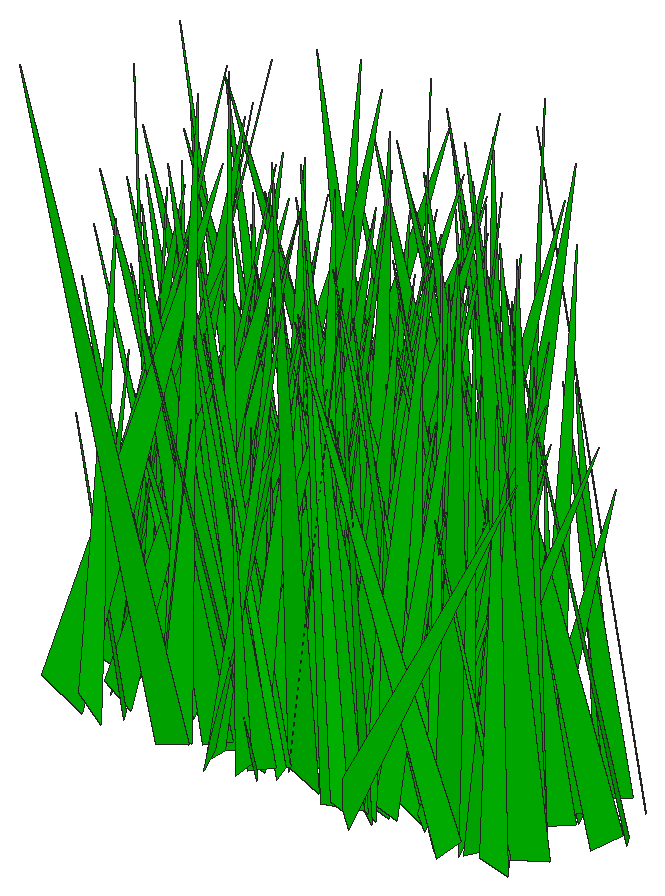
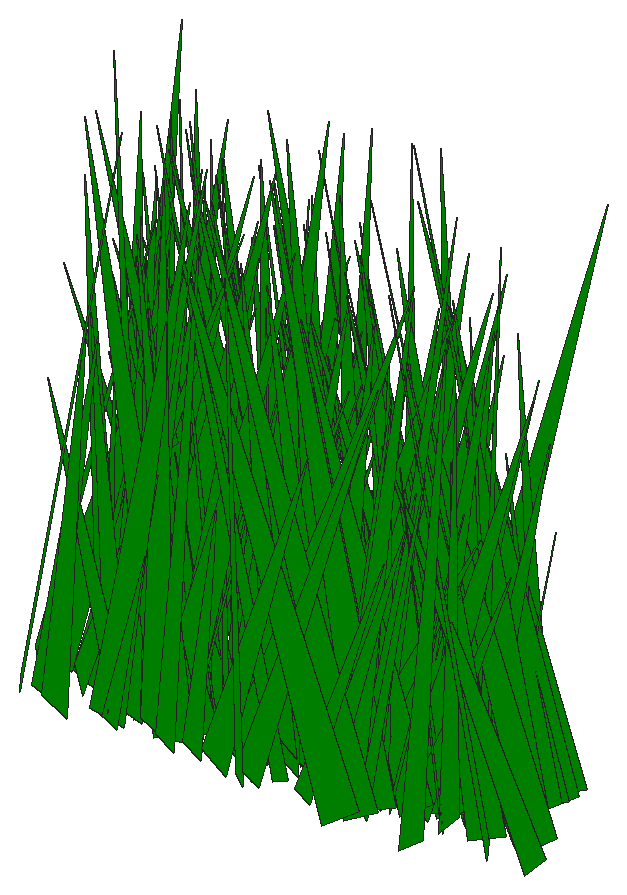
# SketchUp Ruby script. Lengths in inches.
U = 1.inch
M = Sketchup.active_model
def pt(a) = Geom::Point3d.new(a.map { |v| v * U })
def face(e, loops, mat)
  f = e.add_face(loops[0].map { |a| pt(a) })
  loops[1..].each { |l| e.add_face(l.map { |a| pt(a) }).erase! }
  f.material = f.back_material = mat if mat
  f
end
# faces: each face lists its corners as indices into pts; further lists are holes
def faces(e, pts, list, mat = nil) = list.each { |f| face(e, (f[0].is_a?(Array) ? f : [f]).map { |l| l.map { |i| pts[i] } }, mat) }
# xy, xz, yz: faces in a plane at the given z, y or x. An outline is a flat list of corners, or four numbers for a rectangle; further outlines are holes
def ring(l) = l.size == 4 ? [[l[0], l[1]], [l[2], l[1]], [l[2], l[3]], [l[0], l[3]]] : l.each_slice(2).to_a
def flat(e, list, mat, &to3) = list.each { |f| face(e, (f[0].is_a?(Array) ? f : [f]).map { |l| ring(l).map { |u, v| to3.(u, v) } }, mat) }
def xy(e, z, list, mat = nil) = flat(e, list, mat) { |x, y| [x, y, z] }
def xz(e, y, list, mat = nil) = flat(e, list, mat) { |x, z| [x, y, z] }
def yz(e, x, list, mat = nil) = flat(e, list, mat) { |y, z| [x, y, z] }
def lines(e, pts, list) = list.each { |a, b| e.add_line(pt(pts[a]), pt(pts[b])) }
# prism: a flat outline (further loops are holes) pulled along v
def prism(e, loops, v, mat = nil)
  f = face(e, loops, mat); d = Geom::Vector3d.new(v.map { |x| x * U })
  f.pushpull(f.normal.samedirection?(d) ? d.length : -d.length)
end
def box(e, o, s, mat = nil) = prism(e, [[o, [o[0] + s[0], o[1], o[2]], [o[0] + s[0], o[1] + s[1], o[2]], [o[0], o[1] + s[1], o[2]]]], [0, 0, s[2]], mat)
def at(x, y, z, deg = 0) = Geom::Transformation.translation(pt([x, y, z])) * Geom::Transformation.rotation(ORIGIN, Z_AXIS, deg.degrees)
def axes(o, x, y, z) = Geom::Transformation.new([*x, 0, *y, 0, *z, 0, *pt(o).to_a, 1])
def part(name) = M.definitions.add(name)
# library, detail: a bought-in or finely detailed component or shape, given as its bounding box
def library(name, o, s) = part(name).tap { |d| box(d.entities, o, s) }
def detail(e, o, s) = box(e.add_group.entities, o, s)
def put(e, d, t, mat = nil) = e.add_instance(d, t).tap { |i| i.material = mat if mat }
def group(e, t, mat = nil) = e.add_group.tap { |g| g.transformation = t; g.material = mat if mat }.entities
root = M.entities
M.materials.add("[Color G06]").color = [0, 204, 0]
c1 = part("fur_instance\#9")
p = [[0.8125,0,1.79],[0.67,-0.02,1.48],[0,-0.11,0],[0,0.11,0]]
faces(c1.entities,p,[[0,1,2,3]])
put(root,c1,axes([26.27,17.6875,4.28],[1.77503,-0.43818,1.91924],[-2.78158,-0.30358,-2.21547],[-1.94577,0.03424,4.91795]),"[Color G06]")
put(root,c1,axes([25.45,18.56,4.28],[4.99824,-0.16607,3.33353],[-0.63671,-0.74948,-2.15665],[-2.44698,-0.1442,7.37031]),"[Color G06]")
put(root,c1,axes([22.9,19.63,4.28],[2.96113,-0.41722,0.08202],[-2.68322,-0.36541,2.85818],[1.32498,0.19245,5.60482]),"[Color G06]")
put(root,c1,axes([27.2,19.07,4.28],[-1.54116,-0.61948,0.49557],[-4.26601,0.19114,-2.18785],[-1.28316,0.10858,6.67853]),"[Color G06]")
put(root,c1,axes([25.84,19.31,4.28],[-3.96562,0.38661,0.70973],[2.43463,0.52909,-2.72106],[1.40878,0.17392,6.70031]),"[Color G06]")
put(root,c1,axes([26.89,19.16,4.28],[-0.52699,-0.39708,0.70176],[-2.58056,0.03503,-2.05172],[-1.29225,0.09198,3.811]),"[Color G06]")
put(root,c1,axes([26.34,16.33,4.28],[-2.62712,-0.05537,0.68032],[-0.51987,0.35151,-1.19773],[0.3076,0.12115,3.78609]),"[Color G06]")
put(root,c1,axes([24.11,18.14,4.28],[2.16447,-0.64237,0.1245],[-4.56425,-0.2972,1.09648],[0.62903,0.05391,7.52764]),"[Color G06]")
put(root,c1,axes([25.19,16.5,4.28],[2.70805,0.30168,0.39465],[2.03734,-0.37126,1.3736],[-0.77423,0.07826,4.99494]),"[Color G06]")
put(root,c1,axes([25.5,16.09,4.28],[-3.84473,0.4154,1.17109],[2.44382,0.51774,-3.17502],[1.87511,0.17699,6.53922]),"[Color G06]")
put(root,c1,axes([23.45,18.68,4.28],[1.02615,-0.6579,0.47878],[-4.28554,-0.11006,3.14436],[1.99903,0.10178,6.49515]),"[Color G06]")
put(root,c1,axes([25.9375,20.67,4.28],[-3.70608,-0.57537,0.03348],[-3.88339,0.4878,2.7732],[1.39454,-0.17071,7.8115]),"[Color G06]")
put(root,c1,axes([24.31,19.71,4.28],[5.31499,0.07245,1.13215],[0.31095,-0.72555,2.07305],[-0.86434,0.1845,7.70759]),"[Color G06]")
put(root,c1,axes([28.03,15.97,4.28],[-3.66144,-0.67876,0.62945],[-4.83462,0.49276,-1.77831],[-0.70484,0.14601,8.92792]),"[Color G06]")
put(root,c1,axes([24.46,16.68,4.28],[2.90062,0.34995,0.36701],[2.50236,-0.39305,-1.12379],[0.31088,-0.10142,5.62135]),"[Color G06]")
put(root,c1,axes([25.41,18.16,4.28],[4.49687,-0.17073,1.75021],[-0.85864,-0.62894,-2.11996],[-1.46053,-0.15592,6.63512]),"[Color G06]")
put(root,c1,axes([25.95,18.68,4.28],[-2.37703,0.33297,1.33662],[2.26974,0.354,-1.11387],[1.16179,-0.01033,4.91088]),"[Color G06]")
put(root,c1,axes([27.375,17.76,4.28],[-4.54947,0.06993,1.36749],[0.87654,0.56578,3.19006],[0.56601,-0.31406,6.05135]),"[Color G06]")
put(root,c1,axes([24.36,16.68,4.28],[-0.65487,0.62361,2.23704],[4.18524,0.17397,-2.83423],[2.1734,-0.1471,6.13181]),"[Color G06]")
put(root,c1,axes([24.71,19.24,4.28],[0.60019,-0.77466,1.03045],[-5.39528,-0.05427,2.333],[1.49261,0.11534,8.01866]),"[Color G06]")
put(root,c1,axes([27.54,19.47,4.28],[-3.42438,-0.0279,0.36076],[-0.25947,0.45943,-1.41956],[0.17601,0.13443,4.92626]),"[Color G06]")
put(root,c1,axes([27.3,18.77,4.28],[0.57422,-0.64696,1.14365],[-4.49813,-0.1069,-1.90191],[-1.37015,0.07981,6.72314]),"[Color G06]")
put(root,c1,axes([24.34,18.8,4.28],[5.95512,0.27848,0.16632],[1.93577,-0.81472,1.87956],[-0.50328,0.16146,9.19741]),"[Color G06]")
put(root,c1,axes([24.26,17.625,4.28],[6.10667,0.17875,1.03682],[1.38375,-0.84191,-1.53103],[-0.45797,-0.16026,9.19926]),"[Color G06]")
put(root,c1,axes([25.86,17.86,4.28],[-0.90875,0.42445,0.57821],[2.87881,0.13741,-1.48109],[1.06173,-0.00929,4.51077]),"[Color G06]")
put(root,c1,axes([25.3125,17.2,4.28],[4.16854,-0.06504,0.77961],[-0.33247,-0.57072,-1.49838],[-0.6157,-0.13215,6.08737]),"[Color G06]")
put(root,c1,axes([26.09,19.32,4.28],[3.48305,0.17186,0.95936],[0.89412,-0.46209,2.25788],[-1.06371,0.17432,5.03924]),"[Color G06]")
put(root,c1,axes([27.15,17.91,4.28],[0.74767,-0.67482,0.03349],[-4.74169,-0.10279,-1.45787],[-0.96737,-0.01774,7.17185]),"[Color G06]")
put(root,c1,axes([27.29,18.67,4.28],[-2.84415,0.12768,0.36978],[0.78047,0.37703,-1.5453],[0.53888,0.12779,4.18973]),"[Color G06]")
put(root,c1,axes([27.29,18.96,4.28],[-1.89683,0.24786,1.64054],[2.08615,0.23568,1.29742],[0.11065,-0.19454,3.66209]),"[Color G06]")
put(root,c1,axes([24.59,16.21,4.28],[1.58891,0.79693,0.09119],[5.46262,-0.20916,-2.6313],[1.68071,-0.07359,8.46598]),"[Color G06]")
put(root,c1,axes([27.9,20.11,4.28],[-3.23169,-0.19871,1.21615],[-1.60974,0.43256,-1.43578],[0.31872,0.16984,5.07973]),"[Color G06]")
put(root,c1,axes([28.99,19.22,4.28],[-2.38445,-0.35832,0.45863],[-2.29156,0.26532,-2.80061],[-1.20243,0.20493,4.42786]),"[Color G06]")
put(root,c1,axes([28.12,19.46,4.28],[-5.64134,0.17742,2.7107],[1.82193,0.76517,2.71669],[1.26048,-0.31196,8.20511]),"[Color G06]")
put(root,c1,axes([25.63,16.95,4.28],[0.79235,0.49285,1.91099],[3.49801,-0.03004,-2.34969],[1.37486,-0.20759,4.87689]),"[Color G06]")
put(root,c1,axes([25.97,18.42,4.28],[4.63417,0.36447,0.19802],[2.55297,-0.63785,1.40507],[-0.57557,0.10529,7.82664]),"[Color G06]")
put(root,c1,axes([29.33,18.28,4.28],[-2.13214,-0.67353,1.27137],[-4.75759,0.25263,-2.44774],[-1.19101,0.19658,7.5017]),"[Color G06]")
put(root,c1,axes([28.49,19.98,4.28],[-3.85908,0.46128,2.08467],[3.54398,0.53508,1.05359],[0.57302,-0.20275,7.52325]),"[Color G06]")
put(root,c1,axes([28.28,19.57,4.28],[-0.4187,-0.42172,1.40295],[-3.09522,0.02663,-1.14395],[-0.66858,0.14083,4.41739]),"[Color G06]")
put(root,c1,axes([28.8125,16.65,4.28],[-0.3633,0.51505,2.97986],[4.01401,-0.03894,1.86635],[-1.22694,-0.27991,5.22354]),"[Color G06]")
put(root,c1,axes([29.05,16.83,4.28],[-1.94836,-0.30928,0.6708],[-2.14021,0.22503,-1.96701],[-0.73499,0.1646,3.94953]),"[Color G06]")
put(root,c1,axes([28,19.26,4.28],[-2.98145,0.478,0.87276],[3.32316,0.42326,-1.27154],[1.02366,0.01814,6.6698]),"[Color G06]")
put(root,c1,axes([29.15,20.14,4.28],[-1.99478,0.35344,0.24427],[2.46487,0.2624,1.34803],[-0.61263,-0.09508,4.62832]),"[Color G06]")
put(root,c1,axes([28.37,17.39,4.28],[-1.54046,0.39655,2.3548],[3.25066,0.19165,1.04269],[0.05044,-0.24018,4.71993]),"[Color G06]")
put(root,c1,axes([26.62,19.12,4.28],[1.68588,-0.68116,1.21395],[-4.92058,-0.21702,1.27575],[0.55544,0.1449,7.61711]),"[Color G06]")
put(root,c1,axes([26.09,18.84,4.28],[0.64378,-0.66188,1.57226],[-4.57015,-0.03192,2.63658],[1.65831,0.169,6.65581]),"[Color G06]")
put(root,c1,axes([29.43,16.76,4.28],[-1.67869,-0.66195,1.29696],[-4.71741,0.19812,-2.02333],[-1.01648,0.17375,7.24821]),"[Color G06]")
put(root,c1,axes([27.16,18.53,4.28],[2.52312,0.37374,2.37265],[3.09117,-0.33559,-1.27023],[-0.38484,-0.2453,5.3528]),"[Color G06]")
put(root,c1,axes([27.29,16.34,4.28],[3.11741,-0.04666,0.9945],[-0.0873,-0.41943,-1.64959],[-0.73968,-0.14717,4.38601]),"[Color G06]")
put(root,c1,axes([25.9,18.75,4.28],[5.33592,-0.04722,0.10687],[-0.2952,-0.70134,-2.67721],[-0.1807,-0.24871,7.52915]),"[Color G06]")
put(root,c1,axes([27.8,16.38,4.28],[4.07862,-0.43283,4.12409],[-3.83337,-0.59985,1.23632],[-1.59809,0.33422,7.55985]),"[Color G06]")
put(root,c1,axes([26.1,18.12,4.28],[1.77823,-0.70489,0.66344],[-4.88648,-0.22018,2.38239],[1.36821,0.12976,7.64629]),"[Color G06]")
put(root,c1,axes([29.05,17.24,4.28],[-2.7445,0.30956,1.26596],[2.36851,0.37078,1.05447],[0.18898,-0.15145,5.16928]),"[Color G06]")
put(root,c1,axes([30.39,19.27,4.28],[-2.19086,-0.68214,0.78376],[-4.68658,0.265,-2.76769],[-1.49699,0.16868,7.51767]),"[Color G06]")
put(root,c1,axes([29.25,17.5,4.28],[0.8851,-0.74485,0.73749],[-5.12278,-0.13806,-2.28429],[-1.59146,0.03014,7.76309]),"[Color G06]")
put(root,c1,axes([29.16,19.41,4.28],[-3.85812,0.26697,0.5241],[1.81964,0.53328,-1.28328],[0.69074,0.08631,6.30793]),"[Color G06]")
put(root,c1,axes([29.52,20.43,4.28],[-2.05626,0.26389,0.47768],[1.86109,0.25822,1.50863],[-0.46871,-0.13239,3.89465]),"[Color G06]")
put(root,c1,axes([29.32,19.12,4.28],[-0.33842,-0.57712,1.68178],[-4.19055,0.01098,-1.45077],[-0.91319,0.16349,6.03421]),"[Color G06]")
put(root,c1,axes([28.32,17.74,4.28],[-5.08781,0.17892,4.41574],[2.09897,0.76839,1.82557],[2.44333,-0.28752,7.62675]),"[Color G06]")
put(root,c1,axes([26.92,19.24,4.28],[-0.71148,0.69976,0.56846],[4.5804,0.11223,-3.06489],[2.08491,-0.00777,6.92734]),"[Color G06]")
put(root,c1,axes([30.46,16.01,4.28],[-4.00709,-0.06664,0.03972],[-0.46749,0.53821,-1.61695],[-0.1027,0.15023,5.81054]),"[Color G06]")
put(root,c1,axes([28.23,18.42,4.28],[-1.30617,-0.59788,0.3137],[-4.10423,0.1829,1.87173],[1.25804,-0.02406,6.43206]),"[Color G06]")
put(root,c1,axes([30.14,19.22,4.28],[-2.69345,-0.30394,0.85614],[-2.24075,0.34787,-1.55979],[-0.24081,0.16258,4.93804]),"[Color G06]")
put(root,c1,axes([26.64,17.93,4.28],[2.98182,-0.50941,0.32587],[-3.40956,-0.37246,2.80587],[1.32946,0.18732,6.46508]),"[Color G06]")
put(root,c1,axes([31.76,20.08,4.28],[-4.20193,-0.55918,0.66354],[-3.87731,0.53498,-3.05628],[-1.1153,0.2469,8.12516]),"[Color G06]")
put(root,c1,axes([29.94,18.89,4.28],[-0.03393,0.66018,0.84274],[4.6719,-0.01109,1.41814],[-0.95158,-0.07799,6.93247]),"[Color G06]")
put(root,c1,axes([31.19,20.47,4.28],[-3.67944,0.39367,0.43445],[2.77427,0.48492,2.00696],[-0.59828,-0.17247,6.63448]),"[Color G06]")
put(root,c1,axes([27.93,19.42,4.28],[3.18664,-0.37625,0.92188],[-2.76626,-0.42853,1.26757],[0.09307,0.14566,6.11055]),"[Color G06]")
put(root,c1,axes([30.54,16.57,4.28],[-0.12759,0.59536,1.89436],[4.27718,-0.0329,1.83146],[-1.24138,-0.17457,6.1156]),"[Color G06]")
put(root,c1,axes([30.35,16.34,4.28],[0.32518,-0.49633,1.99443],[-3.60133,-0.1,-1.54712],[-1.21658,0.16335,5.1129]),"[Color G06]")
put(root,c1,axes([29.37,17.35,4.28],[2.97609,-0.1143,1.48938],[-0.28837,-0.39942,-2.23403],[-1.25768,-0.17888,4.03664]),"[Color G06]")
put(root,c1,axes([27.73,19.8125,4.28],[1.02576,-0.77373,2.33996],[-5.57939,-0.07736,2.52469],[1.45229,0.24928,8.04661]),"[Color G06]")
put(root,c1,axes([30.42,19.02,4.28],[1.14898,-0.50422,2.18737],[-3.60948,-0.2181,-1.5403],[-1.47929,0.14054,5.45728]),"[Color G06]")
put(root,c1,axes([28.64,17.72,4.28],[3.31764,-0.2381,1.54396],[-1.96795,-0.43672,1.7094],[-0.33124,0.20989,5.30815]),"[Color G06]")
put(root,c1,axes([31.17,18.85,4.28],[-4.35462,0.00751,0.65661],[0.18105,0.58306,1.91576],[0.4039,-0.18036,6.22048]),"[Color G06]")
put(root,c1,axes([29.75,17.6875,4.28],[-1.95787,-0.26787,0.39993],[-1.69894,0.26244,1.61409],[0.93551,-0.08399,3.76826]),"[Color G06]")
put(root,c1,axes([30.85,16.44,4.28],[-3.82385,0.08204,1.11614],[0.76674,0.5213,1.46597],[0.56208,-0.153,5.59336]),"[Color G06]")
put(root,c1,axes([30.04,16.07,4.28],[2.175,-0.29274,0.0888],[-1.86463,-0.27466,-1.99676],[-0.96636,-0.12891,4.05272]),"[Color G06]")
put(root,c1,axes([28.26,18.49,4.28],[0.64794,-0.55134,0.81799],[-3.59703,-0.04714,2.71467],[1.7302,0.10847,5.33739]),"[Color G06]")
put(root,c1,axes([27.79,20.32,4.28],[2.71311,0.7293,1.13449],[5.09515,-0.32938,-2.89429],[1.40309,-0.21412,8.31657]),"[Color G06]")
put(root,c1,axes([29.15,17.02,4.28],[4.92569,0.09177,1.42904],[0.36199,-0.67375,2.18319],[-1.10286,0.18873,7.09911]),"[Color G06]")
put(root,c1,axes([29.52,19.2,4.28],[-2.03805,0.73439,3.1362],[5.4241,0.34303,-1.35378],[1.6487,-0.22073,8.33069]),"[Color G06]")
put(root,c1,axes([31.88,18.26,4.28],[-3.95082,0.06933,0.02048],[0.49145,0.54176,1.07839],[-0.07672,-0.10006,5.85285]),"[Color G06]")
put(root,c1,axes([31.33,18.48,4.28],[-3.74341,-0.01476,0.77574],[0.03513,0.50851,1.49038],[0.52856,-0.13836,5.39496]),"[Color G06]")
put(root,c1,axes([30.23,17.23,4.28],[-3.68005,0.61034,1.01033],[4.06812,0.51429,-2.59094],[1.75069,0.0879,8.14441]),"[Color G06]")
put(root,c1,axes([29.14,16.14,4.28],[4.5273,-0.29597,0.31509],[-2.01405,-0.61591,-1.8187],[-0.70215,-0.14167,7.2484]),"[Color G06]")
put(root,c1,axes([31.57,19.2,4.28],[-1.91815,-0.58028,1.76309],[-4.29731,0.23523,-1.54965],[-0.49132,0.20802,6.67071]),"[Color G06]")
put(root,c1,axes([28.9,16.95,4.28],[1.08763,-0.50144,1.21512],[-3.49586,-0.10273,2.11956],[1.1709,0.15907,5.19948]),"[Color G06]")
put(root,c1,axes([29.65,19.25,4.28],[-0.69831,0.67708,0.74803],[4.73771,0.11099,-1.66087],[1.17506,-0.04511,7.14101]),"[Color G06]")
put(root,c1,axes([28.82,18.31,4.28],[1.84848,0.81729,1.76902],[5.90014,-0.22129,-2.02708],[0.97003,-0.21146,8.95859]),"[Color G06]")
put(root,c1,axes([29.01,18.64,4.28],[3.85435,0.43261,1.83876],[3.33484,-0.50953,-1.84361],[-0.13114,-0.24225,7.16135]),"[Color G06]")
put(root,c1,axes([28.8,17.97,4.28],[1.57566,0.5579,1.15433],[3.91499,-0.17526,-2.20642],[1.12977,-0.17076,6.03598]),"[Color G06]")
put(root,c1,axes([29.9375,16.45,4.28],[-0.94818,0.5218,0.797],[3.62725,0.14717,-1.42971],[1.063,-0.03676,5.58948]),"[Color G06]")
put(root,c1,axes([30.77,19.44,4.28],[2.36754,-0.41677,0.4463],[-2.71632,-0.31971,-2.10941],[-1.28197,-0.09226,5.29381]),"[Color G06]")
put(root,c1,axes([29.18,15.89,4.28],[5.70877,0.32434,0.24955],[2.10431,-0.74305,3.40985],[-1.0048,0.28657,8.55892]),"[Color G06]")
put(root,c1,axes([32.26,20.45,4.28],[-0.38289,0.52583,0.72962],[3.45221,0.0194,2.44095],[-1.59377,-0.08431,5.11196]),"[Color G06]")
put(root,c1,axes([28.13,20.69,4.28],[2.02905,-0.7612,0.02257],[-5.00979,-0.25878,3.46459],[2.16804,0.11444,7.98465]),"[Color G06]")
put(root,c1,axes([32.09,18.91,4.28],[-0.93518,-0.46611,0.84899],[-3.27244,0.10259,-1.58193],[-0.88711,0.11294,4.94055]),"[Color G06]")
put(root,c1,axes([30.32,17.97,4.28],[3.28806,-0.21802,0.07824],[-1.39252,-0.41565,-2.33218],[-0.71289,-0.1937,4.91644]),"[Color G06]")
put(root,c1,axes([32.98,19.09,4.28],[-3.30916,0.35905,0.24395],[2.49667,0.43632,1.8805],[-0.65037,-0.15191,5.97775]),"[Color G06]")
put(root,c1,axes([31.43,16.53,4.28],[-3.5393,-0.63851,1.24748],[-4.46802,0.50706,1.49758],[1.30373,0.00436,8.51892]),"[Color G06]")
put(root,c1,axes([31.18,18.67,4.28],[-2.97514,-0.49726,2.10874],[-3.54612,0.45153,1.05559],[1.46016,0.08337,6.86024]),"[Color G06]")
put(root,c1,axes([31.81,17.26,4.28],[-2.89259,0.20273,2.35451],[1.9911,0.39079,1.59863],[0.79434,-0.24132,4.56681]),"[Color G06]")
put(root,c1,axes([31.32,17.21,4.28],[-2.96996,0.62724,1.10041],[4.34293,0.42662,-1.75229],[1.38346,0.00729,7.86307]),"[Color G06]")
put(root,c1,axes([31.2,19.49,4.28],[3.98199,-0.05528,2.32859],[-0.14583,-0.59036,-1.05285],[-1.60104,-0.08371,5.8874]),"[Color G06]")
put(root,c1,axes([30.16,17.74,4.28],[-0.01629,-0.70521,2.22574],[-5.07177,0.05878,2.05637],[1.43892,0.19919,7.27333]),"[Color G06]")
put(root,c1,axes([32.74,18.54,4.28],[-0.04163,-0.77445,4.17386],[-6.05089,-0.08421,-1.92982],[-1.42486,0.38025,8.07332]),"[Color G06]")
put(root,c1,axes([33.18,17.9375,4.28],[-4.15553,0.04083,0.10108],[0.29869,0.54682,2.05589],[-0.03302,-0.19199,5.87692]),"[Color G06]")
put(root,c1,axes([30.95,19.43,4.28],[-2.36603,0.5596,2.01199],[3.89997,0.3718,-1.63458],[1.64527,-0.07656,6.76803]),"[Color G06]")
put(root,c1,axes([29.14,19.47,4.28],[3.39302,-0.63952,1.39082],[-4.55729,-0.41515,2.90547],[1.06311,0.26144,8.01605]),"[Color G06]")
put(root,c1,axes([30.8125,17.21,4.28],[-1.06045,0.48876,0.15568],[3.28886,0.1439,-1.85412],[1.21627,0.03704,5.14937]),"[Color G06]")
put(root,c1,axes([30.51,17.2,4.28],[4.97512,-0.06874,1.53091],[-0.00688,-0.64306,-3.26679],[-1.13672,-0.29695,6.72014]),"[Color G06]")
put(root,c1,axes([32.97,17.37,4.28],[-3.85192,0.20658,0.68841],[1.54228,0.52849,1.05885],[0.16764,-0.11549,6.07649]),"[Color G06]")
put(root,c1,axes([31.24,20.74,4.28],[5.51857,-0.10881,2.90851],[-0.40345,-0.8049,-1.74927],[-2.05748,-0.13402,8.14422]),"[Color G06]")
put(root,c1,axes([30.84,17.55,4.28],[5.33659,0.39926,0.71394],[2.51268,-0.70518,3.34803],[-1.45344,0.24686,8.40941]),"[Color G06]")
put(root,c1,axes([31.67,18.62,4.28],[-2.86135,0.43223,0.06751],[2.77901,0.36145,-2.7377],[1.37363,0.1691,5.67932]),"[Color G06]")
put(root,c1,axes([33.63,19.69,4.28],[-4.9183,-0.19176,0.08696],[-1.3024,0.65814,2.1723],[0.44511,-0.19311,7.31702]),"[Color G06]")
put(root,c1,axes([32.04,18.12,4.28],[2.46402,0.78891,0.03943],[5.54897,-0.33778,1.78162],[-1.10325,0.06307,9.04901]),"[Color G06]")
put(root,c1,axes([30.4,18.73,4.28],[5.40066,0.08305,1.08432],[0.75741,-0.73455,-1.96356],[-0.55445,-0.19448,7.87965]),"[Color G06]")
put(root,c1,axes([32.9,16.1,4.28],[-0.33592,0.79165,1.34305],[5.70341,0.03033,1.13249],[-0.71319,-0.13029,8.42397]),"[Color G06]")
put(root,c1,axes([33.85,17.89,4.28],[-2.16807,0.37822,0.25159],[2.58745,0.27812,1.7763],[-0.8307,-0.12083,4.87621]),"[Color G06]")
put(root,c1,axes([31.39,18.25,4.28],[4.47109,-0.01844,1.69509],[-0.40254,-0.62357,1.59259],[-1.06853,0.15777,6.49283]),"[Color G06]")
put(root,c1,axes([30.69,18.88,4.28],[1.60078,-0.69015,0.98508],[-4.887,-0.19679,1.90104],[1.02323,0.13981,7.53833]),"[Color G06]")
put(root,c1,axes([32.91,16.01,4.28],[-4.49008,0.28975,1.59695],[1.92592,0.64172,-1.27943],[1.32288,0.0492,7.28295]),"[Color G06]")
put(root,c1,axes([30.44,20.14,4.28],[5.42924,0.36766,1.23171],[2.7443,-0.74684,-1.41164],[-0.31576,-0.16916,8.90949]),"[Color G06]")
put(root,c1,axes([34.36,19.44,4.28],[-0.42866,0.6766,3.05207],[4.89134,-0.05443,2.92065],[-1.94612,-0.28583,6.66845]),"[Color G06]")
put(root,c1,axes([33.54,16.7,4.28],[0.32977,-0.62462,0.98543],[-4.32708,-0.07061,-1.90696],[-1.33253,0.07471,6.43628]),"[Color G06]")
put(root,c1,axes([33.05,20.33,4.28],[0.78509,0.37795,0.13886],[2.54595,-0.10736,1.41507],[-0.93426,0.02503,3.97286]),"[Color G06]")
put(root,c1,axes([30.34,18.87,4.28],[3.33199,0.64013,1.59754],[4.59816,-0.40135,-2.94807],[1.03574,-0.27751,7.94863]),"[Color G06]")
put(root,c1,axes([31.92,17.78,4.28],[0.1813,-0.65482,0.61834],[-4.63911,-0.01453,1.27128],[0.83755,0.06129,6.90762]),"[Color G06]")
put(root,c1,axes([31.81,18.15,4.28],[4.32983,-0.29876,2.0366],[-2.40371,-0.60333,1.24795],[-0.81817,0.19143,7.1115]),"[Color G06]")
put(root,c1,axes([34.2,19.44,4.28],[-2.79779,-0.53345,1.67622],[-3.98475,0.36848,-1.38545],[-0.11962,0.20221,6.94663]),"[Color G06]")
put(root,c1,axes([33.46,18.63,4.28],[-3.34821,-0.22257,0.77622],[-1.37029,0.45579,1.80991],[0.96931,-0.12446,5.23987]),"[Color G06]")
put(root,c1,axes([34.68,18.41,4.28],[-3.70191,0.24795,0.90694],[1.86924,0.46724,2.36925],[-0.1892,-0.23522,5.66221]),"[Color G06]")
put(root,c1,axes([33.22,18.9375,4.28],[1.99986,0.32504,0.95131],[2.17639,-0.29236,1.25533],[-1.04967,0.01309,4.41527]),"[Color G06]")
put(root,c1,axes([33.14,19.3,4.28],[-2.13499,-0.32644,0.84949],[-2.2072,0.30751,1.1833],[0.96518,-0.01888,4.5851]),"[Color G06]")
put(root,c1,axes([33.58,16.16,4.28],[-4.11627,-0.27086,1.90278],[-1.75071,0.59927,1.33966],[1.52603,-0.0431,6.6694]),"[Color G06]")
put(root,c1,axes([33.8,20.44,4.28],[-4.26304,0.20034,3.17662],[2.0878,0.60496,1.87564],[1.49089,-0.27431,6.45661]),"[Color G06]")
put(root,c1,axes([32.95,19.13,4.28],[3.21872,0.25551,0.78041],[1.65193,-0.44547,1.5358],[-0.94937,0.09115,5.31819]),"[Color G06]")
put(root,c1,axes([35.21,19.32,4.28],[0.29509,-0.82608,1.39265],[-5.60375,-0.08431,-3.09264],[-2.13548,0.10709,8.3079]),"[Color G06]")
put(root,c1,axes([32.48,17.58,4.28],[1.97003,-0.4022,1.17352],[-2.9795,-0.25362,1.18746],[0.24121,0.15209,5.0835]),"[Color G06]")
put(root,c1,axes([34.37,16.99,4.28],[-3.64583,-0.43159,0.28071],[-2.9846,0.49941,1.61825],[0.84073,-0.09868,6.96207]),"[Color G06]")
put(root,c1,axes([32.86,19.49,4.28],[2.81404,-0.03444,0.44387],[-0.1152,-0.3655,-1.62658],[-0.3687,-0.14867,3.89604]),"[Color G06]")
put(root,c1,axes([35.27,16.86,4.28],[-4.74583,0.15769,1.03725],[1.26044,0.64809,1.56353],[0.41448,-0.16525,7.12198]),"[Color G06]")
put(root,c1,axes([33.67,16.16,4.28],[-2.38177,0.18656,1.5003],[1.14563,0.35943,-1.07164],[1.21863,0.02672,3.93972]),"[Color G06]")
put(root,c1,axes([36.08,16.05,4.28],[-3.82431,0.39735,0.7504],[2.79644,0.4778,2.77058],[-0.74276,-0.24697,6.56738]),"[Color G06]")
put(root,c1,axes([32.2,17.98,4.28],[4.5786,-0.41105,1.0738],[-3.03148,-0.62722,1.29235],[-0.1243,0.15581,8.03534]),"[Color G06]")
put(root,c1,axes([35.62,16.14,4.28],[-3.75078,-0.13361,0.40536],[-0.98552,0.47693,-2.31092],[-0.14272,0.218,5.30429]),"[Color G06]")
put(root,c1,axes([34.3,20.13,4.28],[2.63594,0.69887,1.3629],[4.85243,-0.38805,1.89497],[-1.55032,-0.02633,8.24845]),"[Color G06]")
put(root,c1,axes([35.76,20.36,4.28],[-4.26756,-0.52819,1.67155],[-3.94576,0.5801,-1.44501],[0.17035,0.20478,8.40483]),"[Color G06]")
put(root,c1,axes([34.2,16.9,4.28],[-3.12156,0.46064,0.87858],[3.04532,0.43597,-2.08879],[1.40844,0.07827,6.46358]),"[Color G06]")
put(root,c1,axes([33.41,16.55,4.28],[-2.05248,0.58128,2.97768],[4.2464,0.35712,-1.47041],[1.82048,-0.17766,6.78698]),"[Color G06]")
put(root,c1,axes([33.25,17.86,4.28],[4.39948,0.38249,2.51323],[3.08213,-0.61501,-1.29966],[-0.92307,-0.23048,7.63889]),"[Color G06]")
put(root,c1,axes([35.29,19.89,4.28],[-4.84612,0.31027,2.32805],[2.51579,0.68021,1.28419],[1.0236,-0.20289,7.86566]),"[Color G06]")
put(root,c1,axes([36.49,19,4.28],[-4.56421,-0.49382,1.65372],[-3.68841,0.57748,-2.92984],[-0.40121,0.30887,8.12177]),"[Color G06]")
put(root,c1,axes([33.5625,20.14,4.28],[2.11123,0.50846,3.17713],[4.21873,-0.26434,-1.40232],[-0.12895,-0.32352,6.13909]),"[Color G06]")
put(root,c1,axes([35.7,20.33,4.28],[-3.09254,0.62991,1.20241],[4.58571,0.41973,1.08571],[-0.1554,-0.14959,8.10959]),"[Color G06]")
put(root,c1,axes([33.36,17.06,4.28],[1.19388,-0.37688,0.6864],[-2.69055,-0.14768,1.13861],[0.52594,0.10004,4.26666]),"[Color G06]")
put(root,c1,axes([33.83,18.55,4.28],[5.6178,0.37352,1.16719],[1.98344,-0.70681,4.65937],[-1.96239,0.35491,8.05071]),"[Color G06]")
put(root,c1,axes([34.24,18.54,4.28],[-2.50144,0.55353,0.76516],[3.71202,0.35233,-2.17245],[1.49657,0.05128,6.66739]),"[Color G06]")
put(root,c1,axes([33.62,19.52,4.28],[3.9271,-0.29211,0.29394],[-1.97659,-0.5321,-1.75669],[-0.7211,-0.13231,6.41602]),"[Color G06]")
put(root,c1,axes([37.42,19.29,4.28],[-5.48146,-0.24789,0.22383],[-1.70292,0.70695,-3.21485],[-0.53163,0.29139,7.98998]),"[Color G06]")
put(root,c1,axes([36.48,17.32,4.28],[-4.72833,-0.25871,2.00013],[-2.27729,0.57296,-3.51187],[0.21689,0.37586,6.73021]),"[Color G06]")
put(root,c1,axes([34.83,17.8,4.28],[3.0471,-0.51654,1.51867],[-3.60998,-0.4469,-1.28217],[-1.31235,0.02998,7.05314]),"[Color G06]")
put(root,c1,axes([33.29,19.41,4.28],[1.82444,-0.44899,0.05241],[-3.06438,-0.24038,1.72685],[0.98887,0.08347,5.25459]),"[Color G06]")
put(root,c1,axes([32.94,18.9,4.28],[3.22465,0.68652,0.77594],[4.88898,-0.42805,-1.87918],[0.77799,-0.1556,8.59286]),"[Color G06]")
put(root,c1,axes([35.57,20.3125,4.28],[-3.03787,0.03453,1.32996],[0.60085,0.39785,1.87909],[0.70153,-0.19122,4.14975]),"[Color G06]")
put(root,c1,axes([36.93,17.68,4.28],[-1.83539,0.55145,0.61387],[3.74202,0.21828,2.46652],[-1.34353,-0.1454,6.03115]),"[Color G06]")
put(root,c1,axes([35.01,16.8,4.28],[-4.56122,0.24607,2.73011],[1.4577,0.6824,-1.62532],[2.07983,0.06137,7.12645]),"[Color G06]")
put(root,c1,axes([33.84,16.52,4.28],[4.50439,-0.29697,1.83538],[-2.35217,-0.62455,1.28606],[-0.71471,0.18382,7.33477]),"[Color G06]")
put(root,c1,axes([34.48,17.76,4.28],[2.96841,0.10265,0.7797],[0.57561,-0.40808,1.27695],[-0.69482,0.10049,4.38891]),"[Color G06]")
put(root,c1,axes([36.37,18.125,4.28],[-0.22876,-0.77959,2.0888],[-5.62086,-0.01282,-1.92482],[-1.27072,0.19706,8.13812]),"[Color G06]")
put(root,c1,axes([33.9,20.03,4.28],[2.80821,-0.63835,3.0945],[-5.02016,-0.34321,2.04335],[0.202,0.34484,7.7621]),"[Color G06]")
put(root,c1,axes([32.79,17.69,4.28],[2.80154,-0.51277,0.61991],[-3.4053,-0.32884,3.12987],[1.44839,0.2187,6.15956]),"[Color G06]")
put(root,c1,axes([35.01,18.5,4.28],[5.08172,-0.27589,2.36546],[-1.55174,-0.72991,-2.33303],[-2.00286,-0.13449,7.80927]),"[Color G06]")
put(root,c1,axes([35.7,18.6875,4.28],[-3.93476,0.46071,0.21232],[2.94765,0.50258,-3.2537],[1.49898,0.22104,6.95552]),"[Color G06]")
put(root,c1,axes([35.05,19.84,4.28],[5.47484,0.25996,3.6652],[2.40909,-0.79594,-1.55311],[-1.91983,-0.25743,8.50326]),"[Color G06]")
put(root,c1,axes([32.97,16.02,4.28],[4.10143,0.31754,0.31011],[1.97394,-0.46169,-4.00816],[1.15423,-0.33879,5.75271]),"[Color G06]")
put(root,c1,axes([36.13,19.18,4.28],[2.11155,-0.6502,1.38052],[-4.55502,-0.31707,-1.59214],[-1.35879,0.05249,7.4826]),"[Color G06]")
put(root,c1,axes([35.43,18.71,4.28],[-1.68865,-0.57466,1.57525],[-4.08261,0.26335,1.26009],[1.19411,0.08773,6.53581]),"[Color G06]")
put(root,c1,axes([34.76,16.68,4.28],[2.87657,-0.07471,0.56266],[-0.65136,-0.35073,2.08869],[-0.06716,0.20161,3.84214]),"[Color G06]")
put(root,c1,axes([35.81,18.52,4.28],[3.37446,0.3634,1.45678],[2.36733,-0.48725,1.71383],[-1.46199,0.0498,6.13753]),"[Color G06]")
put(root,c1,axes([35.6,16.74,4.28],[-2.5225,-0.72557,0.6702],[-4.98579,0.35524,2.26157],[1.5545,-0.03802,8.34111]),"[Color G06]")
put(root,c1,axes([36.54,19.05,4.28],[0.73936,-0.64408,0.60988],[-4.53714,-0.11238,-1.34681],[-0.95648,0.0352,6.86017]),"[Color G06]")
put(root,c1,axes([37.28,18.5,4.28],[-0.29141,0.73515,0.13234],[5.10579,0.03626,1.977],[-1.31623,-0.02212,7.63973]),"[Color G06]")
put(root,c1,axes([35.46,16.97,4.28],[1.93189,0.32965,1.62278],[2.59985,-0.25125,-1.05062],[-0.09089,-0.17992,4.44032]),"[Color G06]")
put(root,c1,axes([37.27,19.21,4.28],[-0.57247,-0.47888,0.21751],[-3.31579,0.07152,-1.40612],[-0.90579,0.04086,5.0099]),"[Color G06]")
put(root,c1,axes([36.0625,19.42,4.28],[-1.89373,0.47698,0.83437],[3.26332,0.27527,-1.5329],[1.16733,0.00425,5.63883]),"[Color G06]")
put(root,c1,axes([35.83,18.01,4.28],[2.50208,0.15268,0.20118],[1.02613,-0.3392,1.0646],[-0.40495,0.08384,3.94064]),"[Color G06]")
put(root,c1,axes([35.1875,17.45,4.28],[4.06383,-0.30738,1.5256],[-2.39952,-0.55118,1.52015],[-0.37863,0.19388,6.74039]),"[Color G06]")
put(root,c1,axes([36.08,16.69,4.28],[5.39686,-0.31837,1.4782],[-1.56564,-0.69054,-4.31692],[-1.93384,-0.32944,7.62028]),"[Color G06]")
put(root,c1,axes([37.54,16.4,4.28],[-3.19181,-0.02873,0.461],[-0.0943,0.42322,1.57107],[0.35873,-0.14434,4.51478]),"[Color G06]")
put(root,c1,axes([36.91,18.93,4.28],[-2.71085,0.26209,0.90169],[1.75668,0.38549,-1.0748],[0.90042,0.03699,4.81157]),"[Color G06]")
put(root,c1,axes([35.45,17.28,4.28],[1.9463,-0.41669,1.57317],[-3.1281,-0.22543,1.78532],[0.50235,0.21067,5.02199]),"[Color G06]")
put(root,c1,axes([36.56,19.07,4.28],[-4.00372,0.53483,1.05988],[3.36827,0.54555,-3.20261],[1.96671,0.15444,7.64257]),"[Color G06]")
put(root,c1,axes([38.69,18.57,4.28],[-0.11142,0.6732,0.42904],[4.31821,-0.00418,3.25865],[-2.17768,-0.04274,6.43977]),"[Color G06]")
put(root,c1,axes([34.57,18.06,4.28],[2.95682,0.42001,0.19831],[2.83065,-0.37781,-2.35333],[1.03796,-0.16614,5.8529]),"[Color G06]")
put(root,c1,axes([38.41,20.32,4.28],[-5.89603,-0.06164,1.33884],[-0.59154,0.81803,-1.49274],[0.80493,0.14967,8.70979]),"[Color G06]")
put(root,c1,axes([37.04,20.71,4.28],[2.0579,-0.48803,0.40482],[-3.27858,-0.28287,-1.94464],[-1.25415,-0.06133,5.74792]),"[Color G06]")
put(root,c1,axes([37.61,20.39,4.28],[0.26105,-0.49126,1.61381],[-3.55187,-0.07372,-1.29444],[-0.98053,0.13624,5.11863]),"[Color G06]")
put(root,c1,axes([35.88,19.6,4.28],[1.0969,0.41197,0.39186],[2.89202,-0.13991,-1.18569],[0.65797,-0.07181,4.55827]),"[Color G06]")
put(root,c1,axes([36.59,16.27,4.28],[3.64185,0.4155,0.94778],[2.81536,-0.51169,1.60444],[-1.16379,0.06239,6.84723]),"[Color G06]")
put(root,c1,axes([39.02,18.91,4.28],[-4.99809,-0.10998,0.41708],[-0.82998,0.68141,-1.57706],[0.10488,0.1515,7.39617]),"[Color G06]")
put(root,c1,axes([37.45,17.1,4.28],[-3.18664,-0.05141,1.85214],[-0.74141,0.44922,-1.41686],[1.05924,0.15975,4.5803]),"[Color G06]")
put(root,c1,axes([37.78,16.8,4.28],[1.72653,-0.7934,2.33548],[-5.70054,-0.28288,-1.62602],[-1.52252,0.15945,8.7365]),"[Color G06]")
put(root,c1,axes([37.3,17.67,4.28],[2.2845,0.48574,1.51088],[3.42705,-0.34363,1.11594],[-1.1879,-0.05721,6.12506]),"[Color G06]")
put(root,c1,axes([37.36,16.09,4.28],[-2.38688,0.49104,0.81725],[3.436,0.34146,-1.1518],[0.94489,-0.00128,6.25282]),"[Color G06]")
put(root,c1,axes([37.69,17.0625,4.28],[2.22541,0.65855,1.85392],[4.6717,-0.34246,1.44799],[-1.42037,-0.09456,7.66723]),"[Color G06]")
